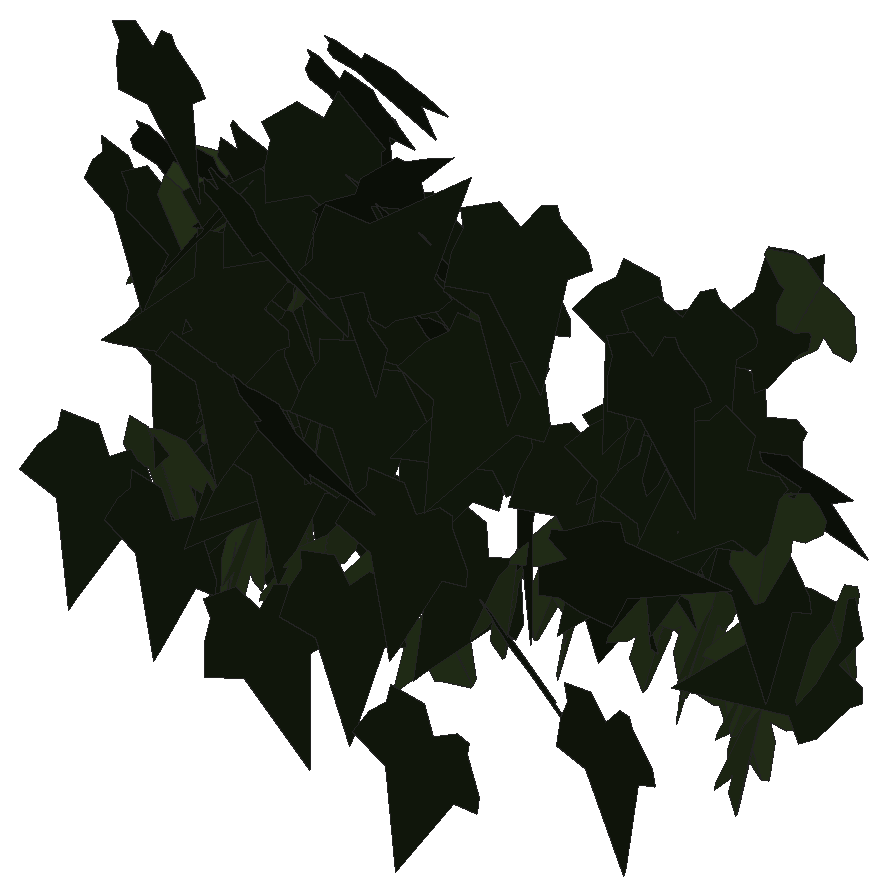
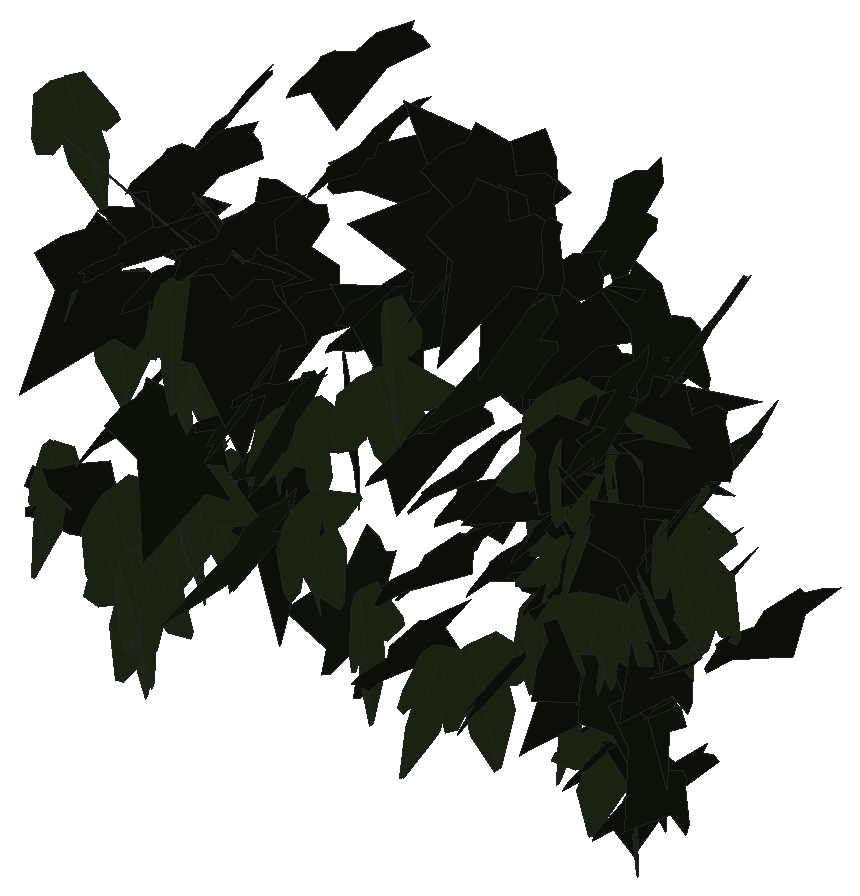
# SketchUp Ruby script. Lengths in inches.
U = 1.inch
M = Sketchup.active_model
def pt(a) = Geom::Point3d.new(a.map { |v| v * U })
def face(e, loops, mat)
  f = e.add_face(loops[0].map { |a| pt(a) })
  loops[1..].each { |l| e.add_face(l.map { |a| pt(a) }).erase! }
  f.material = f.back_material = mat if mat
  f
end
# faces: each face lists its corners as indices into pts; further lists are holes
def faces(e, pts, list, mat = nil) = list.each { |f| face(e, (f[0].is_a?(Array) ? f : [f]).map { |l| l.map { |i| pts[i] } }, mat) }
# xy, xz, yz: faces in a plane at the given z, y or x. An outline is a flat list of corners, or four numbers for a rectangle; further outlines are holes
def ring(l) = l.size == 4 ? [[l[0], l[1]], [l[2], l[1]], [l[2], l[3]], [l[0], l[3]]] : l.each_slice(2).to_a
def flat(e, list, mat, &to3) = list.each { |f| face(e, (f[0].is_a?(Array) ? f : [f]).map { |l| ring(l).map { |u, v| to3.(u, v) } }, mat) }
def xy(e, z, list, mat = nil) = flat(e, list, mat) { |x, y| [x, y, z] }
def xz(e, y, list, mat = nil) = flat(e, list, mat) { |x, z| [x, y, z] }
def yz(e, x, list, mat = nil) = flat(e, list, mat) { |y, z| [x, y, z] }
def lines(e, pts, list) = list.each { |a, b| e.add_line(pt(pts[a]), pt(pts[b])) }
# prism: a flat outline (further loops are holes) pulled along v
def prism(e, loops, v, mat = nil)
  f = face(e, loops, mat); d = Geom::Vector3d.new(v.map { |x| x * U })
  f.pushpull(f.normal.samedirection?(d) ? d.length : -d.length)
end
def box(e, o, s, mat = nil) = prism(e, [[o, [o[0] + s[0], o[1], o[2]], [o[0] + s[0], o[1] + s[1], o[2]], [o[0], o[1] + s[1], o[2]]]], [0, 0, s[2]], mat)
def at(x, y, z, deg = 0) = Geom::Transformation.translation(pt([x, y, z])) * Geom::Transformation.rotation(ORIGIN, Z_AXIS, deg.degrees)
def axes(o, x, y, z) = Geom::Transformation.new([*x, 0, *y, 0, *z, 0, *pt(o).to_a, 1])
def part(name) = M.definitions.add(name)
# library, detail: a bought-in or finely detailed component or shape, given as its bounding box
def library(name, o, s) = part(name).tap { |d| box(d.entities, o, s) }
def detail(e, o, s) = box(e.add_group.entities, o, s)
def put(e, d, t, mat = nil) = e.add_instance(d, t).tap { |i| i.material = mat if mat }
def group(e, t, mat = nil) = e.add_group.tap { |g| g.transformation = t; g.material = mat if mat }.entities
root = M.entities
M.materials.add("efeu1").color = [18, 25, 13]
M.materials.add("efeu2").color = [43, 57, 29]
c1 = part("ivyleaf_10")
p = [[0,0.5,-0.03],[-0.0625,2.02,-0.43],[-0.19,2.01,-0.46],[-0.54,1.05,-0.29],[-0.52,0.625,-0.18],[-0.83,0.76,-0.28],
  [-1.16,0.64,-0.33],[-1.15,0.33,-0.24],[-0.77,-0.39,0.02],[-0.3,-0.51,0.16],[0.04,-0.48,0.23],[-0.02,2.01,-0.4375],
  [-0.06,2.01,-0.43],[0.04,-0.49,0.23],[0.67,-0.49,0.14],[1.38,0.36,-0.2],[1.375,0.51,-0.24],[0.81,0.65,-0.19],
  [0.62,0.59,-0.15],[0.6,1.09,-0.28],[0.5,1.23,-0.31]]
faces(c1.entities,p,[[0,1,2,3,4,5,6,7,8,9,10],[11,12,0,13,14,15,16,17,18,19,20]],"efeu2")
c2 = part("ivyleaf_9")
p = [[1.54,2.16,1.25],[1.36,2.04,1.19],[-0.21,0.99,0.68],[-0.71,1.11,0.82],[-0.85,0.86,0.67],[-0.8,0.17,0.21],
  [-0.9,-0.01,0.1],[-0.67,-0.16,-0.02],[-0.08,-0.08,-0.05],[-0.03,-0.6,-0.4],[0.65,-0.88,-0.66],[0.83,-0.6,-0.49],
  [1.29,-0.42,-0.43],[1.8125,-0.07,-0.26],[1.21,0.44,0.15]]
faces(c2.entities,p,[[0,1,2,3,4,5,6,7,8,9,10,11,12,13,14]],"efeu1")
put(root,c1,axes([21.97,221.89,251.45],[-0.00265,-0.49967,-0.01785],[-0.0185,0.01794,-0.49934],[0.49965,-0.00198,-0.01858]))
put(root,c2,axes([22.08,222.04,249.17],[0.0361,0.31097,0.38986],[-0.02817,0.39153,-0.30969],[-0.4979,0.00039,0.04579]))
put(root,c2,axes([21.81,221.44,252.02],[0.05871,-0.42685,0.25368],[0.08143,-0.24371,-0.42892],[0.48982,0.09168,0.04091]))
put(root,c2,axes([21.92,221.71,251.89],[0.19244,-0.45963,-0.04136],[-0.01062,0.0404,-0.49825],[0.46136,0.19264,0.00579]))
put(root,c2,axes([22.15,221.53,252.52],[0.41781,0.13911,-0.23682],[-0.23085,-0.05569,-0.44001],[-0.14879,0.47702,0.01769]))
put(root,c2,axes([21.98,221.43,253.52],[0.22053,-0.44662,0.04354],[0.01424,-0.04152,-0.49807],[0.44852,0.22091,-0.00559]))
put(root,c2,axes([22.52,221.99,249.76],[-0.143,0.47908,0.00563],[-0.0342,-0.00435,-0.49881],[-0.47789,-0.14304,0.03401]))
put(root,c2,axes([22.15,222.05,248.82],[0.04628,-0.49078,-0.08361],[-0.01349,0.0827,-0.49293],[0.49767,0.04788,-0.00559]))
put(root,c2,axes([22.23,220.42,249.8],[-0.11905,-0.47907,0.07952],[-0.0079,-0.07995,-0.4935],[0.48556,-0.11876,0.01147]))
put(root,c2,axes([22.47,221.43,250.09],[0.02196,0.34343,0.36273],[0.04359,0.36038,-0.34384],[-0.49761,0.04672,-0.01411]))
put(root,c1,axes([22.46,221.71,250.46],[0.00879,-0.46798,0.17582],[0.00457,-0.17577,-0.46806],[0.4999,0.00983,0.00118]))
put(root,c2,axes([22.77,221.95,250.375],[0.15582,0.004,0.47508],[-0.4711,0.066,0.15396],[-0.06148,-0.49561,0.02434]))
put(root,c1,axes([22.48,222.1,249.21],[0.1564,0.44616,0.16272],[0.00445,0.16994,-0.47021],[-0.47489,0.14853,0.04919]))
put(root,c1,axes([22.24,221.61,252.11],[-0.18213,-0.08844,-0.45717],[0.44797,-0.16727,-0.1461],[-0.1271,-0.46281,0.14017]))
put(root,c2,axes([22.49,221.48,250.64],[-0.11898,-0.43862,0.20846],[0.01983,-0.21883,-0.44913],[0.48523,-0.09861,0.06947]))
put(root,c1,axes([22.61,222.01,249.87],[0.08878,-0.45801,0.17985],[0.03737,-0.17596,-0.46652],[0.49063,0.09628,0.00299]))
put(root,c2,axes([22.46,222.08,249.25],[0.10283,-0.4748,-0.1183],[0.00017,0.12092,-0.48516],[0.48931,0.09974,0.02503]))
put(root,c2,axes([22.59,222.03,249.51],[-0.13852,-0.44909,0.17068],[-0.00174,-0.17717,-0.46756],[0.48043,-0.13012,0.04752]))
put(root,c1,axes([22.6875,221.72,248.69],[0.29406,-0.38853,-0.11212],[-0.00241,0.13694,-0.48088],[0.40438,0.28335,0.07866]))
put(root,c1,axes([22.64,221.67,250.7],[0.3872,-0.30279,0.0916],[0.06171,-0.06971,-0.49126],[0.31027,0.39174,-0.01661]))
put(root,c2,axes([22.83,221.97,250.12],[0.04166,0.4509,-0.21203],[-0.02003,-0.21109,-0.45282],[-0.49786,0.04622,0.00047]))
put(root,c1,axes([22.82,222.17,250.41],[-0.48566,-0.11887,0.00189],[-0.0028,0.0035,-0.49998],[0.11886,-0.48565,-0.00406]))
put(root,c2,axes([23.12,221.93,251.03],[0.02255,0.04663,0.49731],[-0.43421,0.24789,-0.00355],[-0.24689,-0.43171,0.05167]))
put(root,c2,axes([22.66,221.9,250.18],[0.39034,0.29941,0.08936],[0.07776,0.04542,-0.49182],[-0.30263,0.39786,-0.0111]))
put(root,c1,axes([22.8,220.5,250.11],[-0.48359,0.10965,-0.06421],[0.06219,-0.01612,-0.49586],[-0.11081,-0.48756,0.00195]))
put(root,c2,axes([23.16,221.65,251.87],[-0.42783,-0.15647,0.20611],[-0.17969,-0.10694,-0.45417],[0.18622,-0.46269,0.03527]))
put(root,c2,axes([23.19,221.7,252.125],[-0.0165,0.35506,-0.35166],[-0.13615,-0.34173,-0.33865],[-0.48082,0.08458,0.10796]))
put(root,c1,axes([22.91,221.57,251.78],[0.10122,-0.27457,0.40542],[0.15207,-0.37589,-0.29254],[0.46543,0.18253,0.00741]))
put(root,c1,axes([23.08,222.16,250.19],[-0.25808,-0.39444,0.16677],[-0.02134,-0.18263,-0.46497],[0.42772,-0.24711,0.07743]))
put(root,c2,axes([22.78,221.71,252.61],[0.3996,-0.26241,-0.14648],[-0.09422,0.12203,-0.47564],[0.28538,0.40774,0.04808]))
put(root,c1,axes([23.07,221.8,251.43],[-0.17511,0.36112,0.29821],[-0.13878,0.26407,-0.40126],[-0.4473,-0.2233,0.00775]))
put(root,c1,axes([23.11,221.34,249.06],[0.43191,-0.24689,-0.04994],[-0.02625,0.05448,-0.49633],[0.25052,0.43137,0.0341]))
put(root,c1,axes([23.18,221.35,249.13],[0.21127,-0.44641,-0.07799],[-0.03899,0.06783,-0.49384],[0.45149,0.21475,-0.00615]))
put(root,c2,axes([23.13,221.53,252.05],[-0.16099,-0.37937,0.28312],[-0.05446,-0.28222,-0.40913],[0.47023,-0.16257,0.04954]))
put(root,c1,axes([23.17,221.89,250.97],[0.08525,0.49156,0.03319],[0.01604,0.03089,-0.49879],[-0.49242,0.08611,-0.0105]))
put(root,c2,axes([23.43,220.25,252.625],[0.04074,0.41049,0.28255],[-0.05535,0.28547,-0.40675],[-0.49525,0.00187,0.0687]))
put(root,c1,axes([23.3,221.84,251.83],[0.0534,-0.4883,0.09336],[0.0499,-0.08816,-0.48963],[0.49463,0.06161,0.03932]))
put(root,c2,axes([23.43,221.77,251.3125],[-0.38637,-0.30465,0.08894],[-0.07872,-0.04375,-0.49182],[0.30745,-0.39405,-0.01416]))
put(root,c2,axes([23.125,220.23,249.54],[0.01753,-0.45979,0.19566],[0.01888,-0.19504,-0.46],[0.49934,0.02352,0.01052]))
put(root,c2,axes([23.29,221.75,251.49],[-0.18397,-0.41735,0.20487],[-0.07551,-0.19058,-0.45605],[0.45875,-0.19874,0.0071]))
put(root,c2,axes([23.4,221.36,249.9375],[-0.14063,-0.36686,0.30925],[-0.11515,-0.28704,-0.39288],[0.46579,-0.18172,-0.00375]))
put(root,c2,axes([23.71,220.76,251.77],[-0.29745,-0.14521,0.37475],[-0.32804,-0.18164,-0.33076],[0.2322,-0.44263,0.01279]))
put(root,c1,axes([23.4,221.82,251.7],[-0.43329,-0.21681,-0.12353],[0.16222,-0.05667,-0.46954],[0.1896,-0.44697,0.11945]))
put(root,c1,axes([23.48,221.59,249.35],[0.1241,-0.43851,-0.20569],[0.03906,0.2207,-0.44695],[0.48278,0.09486,0.08904]))
put(root,c2,axes([23.34,221.92,251.36],[0.03188,-0.49419,0.06897],[0.00222,-0.06897,-0.49522],[0.49898,0.03188,-0.0022]))
put(root,c1,axes([23.58,221.72,252.16],[-0.12769,-0.47619,0.08328],[0.00637,-0.08778,-0.49219],[0.48338,-0.12464,0.02848]))
put(root,c2,axes([23.23,221.73,251.82],[0.48148,-0.05008,0.12519],[0.12519,-0.00644,-0.48403],[0.05009,0.49744,0.00634]))
put(root,c1,axes([23.68,221.68,250.21],[0.26444,-0.34738,-0.24372],[-0.05234,0.25828,-0.42491],[0.42111,0.25024,0.10024]))
put(root,c2,axes([23.82,221.52,250.35],[-0.38409,-0.27708,0.16031],[-0.07142,-0.16991,-0.46479],[0.31204,-0.37994,0.09095]))
put(root,c2,axes([23.64,220.64,251.375],[-0.12125,-0.47341,0.10577],[0.0849,-0.12805,-0.47581],[0.47759,-0.09742,0.11144]))
put(root,c2,axes([23.75,221.23,250.27],[-0.0386,-0.49463,0.06207],[0.00808,-0.06287,-0.49597],[0.49844,-0.03728,0.01284]))
put(root,c2,axes([23.71,221.91,252.99],[0.47042,-0.12598,-0.11329],[-0.05354,0.20666,-0.45213],[0.16075,0.43751,0.18095]))
put(root,c2,axes([23.87,221.03,252.93],[-0.05037,-0.36812,-0.33459],[0.03701,0.33259,-0.3715],[0.49608,-0.06219,-0.00626]))
put(root,c2,axes([23.87,221.93,249.5625],[0.21372,-0.43448,-0.1247],[-0.02013,0.12865,-0.48275],[0.45157,0.21136,0.0375]))
put(root,c2,axes([24.07,221.56,253.89],[0.4326,0.07916,-0.23788],[-0.23617,-0.03055,-0.43965],[-0.08414,0.49275,0.01096]))
put(root,c2,axes([23.93,221.48,253.4375],[0.03049,-0.41092,-0.28322],[0.00769,0.2841,-0.41137],[0.49901,0.02073,0.02364]))
put(root,c2,axes([24.15,221.79,254.03],[0.44269,0.14473,-0.18188],[-0.19915,0.03444,-0.45733],[-0.11985,0.47735,0.08814]))
put(root,c2,axes([24,219.9375,253.39],[0.4404,-0.22488,-0.07399],[-0.04061,0.0822,-0.49152],[0.23323,0.43894,0.05413]))
put(root,c1,axes([24.33,220.92,249.39],[-0.06042,-0.49488,-0.03796],[-0.0007,0.03832,-0.49853],[0.49634,-0.06019,-0.00532]))
put(root,c1,axes([24.5625,221.71,249.07],[-0.08254,-0.48873,0.0658],[-0.00124,-0.06651,-0.49556],[0.49314,-0.08197,0.00977]))
put(root,c2,axes([24.51,221.47,251.03],[-0.08162,-0.48952,-0.06089],[0.00791,0.06041,-0.49627],[0.49323,-0.08197,-0.00212]))
put(root,c2,axes([24.4375,221.4,252.375],[0.0887,-0.48247,0.09674],[0.02317,-0.09409,-0.49052],[0.49152,0.0915,0.00567]))
put(root,c2,axes([24.4375,219.99,251.17],[0.3306,-0.21049,0.31048],[0.25544,-0.17674,-0.39181],[0.27469,0.41768,-0.00933]))
put(root,c2,axes([24.91,222.11,250.25],[-0.14993,-0.45333,0.14836],[-0.00022,-0.15545,-0.47522],[0.47699,-0.14257,0.04641]))
put(root,c2,axes([24.8125,219.4375,249.54],[0.10389,-0.46918,-0.13813],[0.01509,0.14422,-0.47851],[0.48886,0.09525,0.04413]))
put(root,c2,axes([24.86,222,251.62],[0.05642,-0.47391,-0.14907],[-0.00514,0.14947,-0.47711],[0.49678,0.05537,0.012]))
put(root,c2,axes([24.93,221.65,251.8],[0.08467,-0.48987,-0.05349],[-0.00595,0.05325,-0.49712],[0.49274,0.08482,0.00319]))
put(root,c2,axes([25.14,220.46,253.6],[0.22262,0.43291,0.11414],[0.04685,0.10425,-0.48676],[-0.44525,0.22742,0.00585]))
put(root,c1,axes([25.2,221.51,248.73],[-0.01043,-0.44503,-0.22769],[0.11408,0.2196,-0.43446],[0.4867,-0.06102,0.09696]))
put(root,c2,axes([25.3,222.07,249.13],[-0.15068,-0.41886,0.22771],[-0.05368,-0.22239,-0.44459],[0.47372,-0.15843,0.02205]))
put(root,c2,axes([25.2,220.23,249.58],[0.02541,-0.49768,0.0409],[0.00485,-0.0407,-0.49832],[0.49933,0.02572,0.00276]))
put(root,c2,axes([25.19,221.24,252.98],[0.22759,-0.43711,-0.08449],[-0.01117,0.08926,-0.49184],[0.44506,0.22577,0.03087]))
put(root,c1,axes([25.72,221.52,252.27],[0.15648,-0.45065,-0.14977],[-0.02512,0.14961,-0.47643],[0.47422,0.15663,0.02418]))
put(root,c1,axes([25.8,221.59,251.55],[-0.31146,-0.35443,0.16544],[-0.04202,-0.17994,-0.4646],[0.38888,-0.30332,0.0823]))
put(root,c1,axes([25.8,221.83,249.26],[0.11848,-0.47787,-0.08717],[0.00659,0.0913,-0.49155],[0.48571,0.11533,0.02794]))
put(root,c2,axes([25.59,220.01,252.99],[-0.16317,-0.04248,0.47071],[0.47161,0.018,0.16511],[-0.03097,0.49787,0.03419]))
put(root,c2,axes([25.69,220.5625,250.35],[-0.05831,-0.47888,0.13144],[0.03069,-0.13556,-0.48029],[0.49564,-0.04794,0.0452]))
put(root,c2,axes([25.5,220.81,253.03],[0.33709,-0.23946,0.28112],[0.25798,-0.11964,-0.41126],[0.26423,0.42231,0.0429]))
put(root,c2,axes([25.79,221.03,251.83],[0.20233,-0.23779,0.39054],[0.31457,-0.23755,-0.3076],[0.33183,0.37017,0.05348]))
put(root,c1,axes([26.53,221.83,249.93],[-0.00756,-0.44657,0.22477],[0.05564,-0.22415,-0.44346],[0.49684,0.01831,0.05308]))
put(root,c2,axes([26.7,220.84,251.68],[-0.23982,-0.19543,0.3928],[-0.21718,-0.33608,-0.2998],[0.38121,-0.31442,0.07631]))
put(root,c2,axes([26.29,221.26,248.95],[0.31921,-0.31318,0.22367],[0.15101,-0.16536,-0.44705],[0.35398,0.35295,-0.01098]))
put(root,c2,axes([26.56,219.72,248.72],[-0.07577,-0.45641,0.18961],[0.02549,-0.19518,-0.45962],[0.49357,-0.05999,0.05285]))
put(root,c2,axes([26.65,220.98,250.76],[-0.09268,-0.01737,-0.49103],[0.48033,-0.10838,-0.08682],[-0.10342,-0.4878,0.03678]))
put(root,c1,axes([26.9375,221.43,249.76],[0.29169,-0.40588,0.01333],[0.01073,-0.0087,-0.49981],[0.40595,0.29187,0.00364]))
put(root,c2,axes([26.79,222.07,249.91],[0.4071,-0.23487,-0.1706],[-0.0635,0.21468,-0.44708],[0.28326,0.38568,0.14496]))
put(root,c2,axes([27.18,221.41,249.97],[0.32981,0.07375,-0.36849],[-0.35413,-0.1031,-0.33759],[-0.12577,0.48367,-0.01577]))
put(root,c2,axes([26.81,221.68,250.91],[0.31752,-0.38584,0.01742],[0.01105,-0.01347,-0.4997],[0.38608,0.31772,-0.00003]))
put(root,c2,axes([26.93,220.49,253.36],[0.00125,-0.49234,0.08717],[0.01684,-0.08708,-0.49207],[0.49971,0.00416,0.01637]))
put(root,c1,axes([27.1875,221.17,250.49],[-0.20258,-0.45572,0.03574],[0.00211,-0.04002,-0.49839],[0.45712,-0.20178,0.01814]))
put(root,c2,axes([27.26,219.83,252.79],[-0.33218,-0.37361,0.0087],[-0.00084,-0.0109,-0.49988],[0.37371,-0.33211,0.00661]))
put(root,c2,axes([27.27,220.14,254.07],[-0.03591,-0.47763,-0.14347],[0.02356,0.14205,-0.47882],[0.49815,-0.04115,0.0123]))
put(root,c2,axes([27.51,220.89,251.52],[-0.11543,-0.4488,-0.18776],[0.04042,0.18346,-0.46337],[0.48481,-0.12215,-0.00607]))
put(root,c2,axes([27.65,221.47,250.69],[-0.26957,-0.38692,0.16621],[-0.03516,-0.17598,-0.46668],[0.41964,-0.2633,0.06767]))
put(root,c2,axes([27.65,221.71,252.65],[-0.16405,-0.45169,0.13806],[-0.03133,-0.13542,-0.48029],[0.47128,-0.16623,0.01612]))
put(root,c2,axes([27.47,221.48,250.95],[0.3016,-0.39862,-0.01155],[-0.00654,0.00954,-0.49987],[0.39874,0.30167,0.00054]))
put(root,c1,axes([27.81,221.58,249.83],[-0.00718,-0.49757,0.04873],[0.00375,-0.04878,-0.4976],[0.49993,-0.00678,0.00444]))
put(root,c2,axes([27.89,221.23,251.62],[0.21968,0.37321,-0.2499],[-0.14741,-0.20288,-0.43256],[-0.42428,0.26373,0.02089]))
put(root,c1,axes([27.9,221.92,249.93],[-0.36546,-0.3387,-0.0415],[0.02248,0.03677,-0.49814],[0.34049,-0.36596,-0.01165]))
put(root,c2,axes([28.03,221.75,250.4375],[0.11027,0.46214,0.15577],[0.00199,0.15927,-0.47395],[-0.48768,0.10515,0.03328]))
put(root,c1,axes([28.11,221.72,249.59],[0.25443,-0.42936,0.03027],[0.01273,-0.02765,-0.49907],[0.43024,0.25473,-0.00314]))
put(root,c2,axes([28.26,221.21,251.81],[-0.42328,-0.26122,0.051],[-0.04049,-0.0315,-0.49736],[0.26305,-0.42517,0.00551]))
put(root,c2,axes([28.41,220.87,252.25],[-0.45118,0.21316,-0.03154],[0.02686,-0.01699,-0.49899],[-0.2138,-0.45197,0.00388]))
put(root,c1,axes([28.21,221.7,251.7],[0.04866,-0.48714,-0.10162],[0.02581,0.10444,-0.48829],[0.49696,0.04228,0.03531]))
put(root,c1,axes([28.21,221.75,249.95],[-0.00508,-0.46896,0.17336],[0.06934,-0.17235,-0.46421],[0.49514,0.01933,0.06678]))
put(root,c2,axes([28.3,220.91,251.82],[-0.41861,-0.2675,-0.05667],[0.05397,0.02075,-0.49665],[0.26806,-0.42192,0.0115]))
put(root,c1,axes([28.28,222.06,248.86],[-0.49856,0.00738,-0.03719],[0.03699,-0.01271,-0.49847],[-0.00831,-0.49978,0.01213]))
put(root,c1,axes([28.27,221.44,250.97],[0.1359,-0.43518,0.2053],[0.06155,-0.19586,-0.45591],[0.47722,0.14919,0.00034]))
put(root,c1,axes([28.34,222.2,248.85],[0.16088,-0.47298,0.02011],[0.00295,-0.02023,-0.49958],[0.4734,0.16086,-0.00372]))
put(root,c2,axes([28.32,221.35,251.94],[-0.03168,-0.48731,-0.10734],[0.01459,0.1066,-0.48829],[0.49878,-0.03407,0.00746]))
put(root,c1,axes([28.54,221.91,248.6],[0.156,-0.47314,-0.04249],[-0.00167,0.04418,-0.49804],[0.47504,0.15553,0.01221]))
put(root,c2,axes([28.36,221.15,253.07],[0.00693,-0.44596,-0.22599],[0.00398,0.22605,-0.44596],[0.49994,0.00438,0.00668]))
put(root,c1,axes([28.58,222.12,249.49],[-0.06919,-0.45602,0.19303],[0.02563,-0.19794,-0.45844],[0.49453,-0.05354,0.05077]))
put(root,c2,axes([29.05,221.88,253.0625],[-0.42778,0.22218,0.13281],[-0.14885,-0.00125,-0.47733],[-0.21177,-0.44792,0.06721]))
put(root,c2,axes([28.64,220.88,251.6],[-0.13731,-0.4776,0.05521],[-0.00957,-0.0547,-0.49691],[0.48068,-0.13752,0.00588]))
put(root,c2,axes([28.38,219.52,251.33],[0.13676,0.19305,-0.44049],[0.25744,0.35743,0.23657],[0.40623,-0.2915,-0.00163]))
put(root,c2,axes([28.6,220.41,253.07],[0.16816,-0.46954,-0.03543],[-0.0111,0.03366,-0.49874],[0.47074,0.16853,0.0009]))
put(root,c2,axes([28.87,221.64,252.03],[-0.24851,-0.38309,0.20367],[-0.0222,-0.22317,-0.44688],[0.4333,-0.23116,0.09391]))
put(root,c2,axes([28.68,221.84,250.48],[0.07858,-0.48416,0.09704],[0.0134,-0.09613,-0.49049],[0.4936,0.07969,-0.00214]))
put(root,c2,axes([29.31,222.11,249.44],[-0.35716,-0.07083,0.34267],[-0.32595,-0.11075,-0.36262],[0.12727,-0.48241,0.03294]))
put(root,c2,axes([28.78,219.49,249.74],[0.13892,-0.46638,0.11485],[0.0158,-0.11506,-0.48633],[0.48005,0.13875,-0.01722]))
put(root,c2,axes([29.29,220.82,251.99],[-0.43762,-0.21593,0.10894],[-0.09882,-0.04592,-0.48798],[0.22074,-0.44863,-0.00248]))
put(root,c1,axes([29.19,221.37,251.28],[-0.28167,-0.41024,0.04863],[-0.01508,-0.04861,-0.4974],[0.41284,-0.28167,0.01501]))
put(root,c1,axes([29.4375,221.74,253.47],[-0.41906,0.03039,0.27104],[-0.2727,-0.05532,-0.41542],[0.00474,-0.496,0.06294]))
put(root,c2,axes([29.07,221.49,251.66],[0.48451,0.11688,-0.03987],[-0.04306,0.00861,-0.49807],[-0.11574,0.48607,0.01841]))
put(root,c1,axes([29.29,222.14,249.77],[0.04499,-0.4228,-0.2631],[0.01551,0.26523,-0.42357],[0.49773,0.02995,0.03698]))
